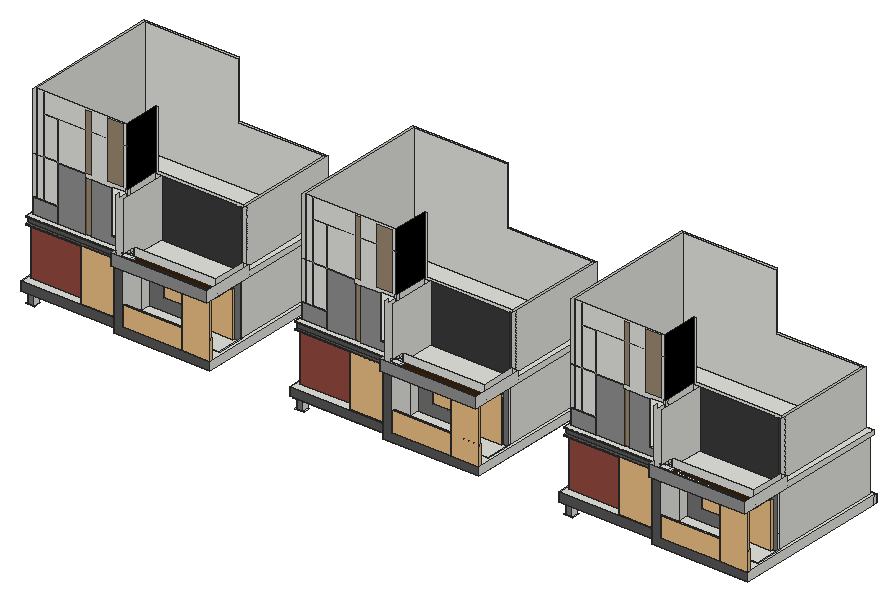
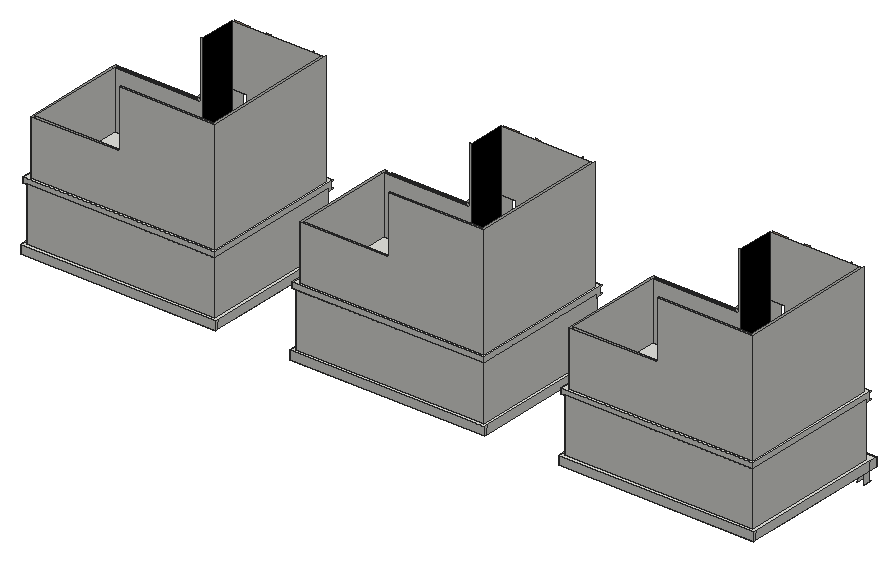
# SketchUp Ruby script. Lengths in inches.
U = 1.inch
M = Sketchup.active_model
def pt(a) = Geom::Point3d.new(a.map { |v| v * U })
def face(e, loops, mat)
  f = e.add_face(loops[0].map { |a| pt(a) })
  loops[1..].each { |l| e.add_face(l.map { |a| pt(a) }).erase! }
  f.material = f.back_material = mat if mat
  f
end
# faces: each face lists its corners as indices into pts; further lists are holes
def faces(e, pts, list, mat = nil) = list.each { |f| face(e, (f[0].is_a?(Array) ? f : [f]).map { |l| l.map { |i| pts[i] } }, mat) }
# xy, xz, yz: faces in a plane at the given z, y or x. An outline is a flat list of corners, or four numbers for a rectangle; further outlines are holes
def ring(l) = l.size == 4 ? [[l[0], l[1]], [l[2], l[1]], [l[2], l[3]], [l[0], l[3]]] : l.each_slice(2).to_a
def flat(e, list, mat, &to3) = list.each { |f| face(e, (f[0].is_a?(Array) ? f : [f]).map { |l| ring(l).map { |u, v| to3.(u, v) } }, mat) }
def xy(e, z, list, mat = nil) = flat(e, list, mat) { |x, y| [x, y, z] }
def xz(e, y, list, mat = nil) = flat(e, list, mat) { |x, z| [x, y, z] }
def yz(e, x, list, mat = nil) = flat(e, list, mat) { |y, z| [x, y, z] }
def lines(e, pts, list) = list.each { |a, b| e.add_line(pt(pts[a]), pt(pts[b])) }
# prism: a flat outline (further loops are holes) pulled along v
def prism(e, loops, v, mat = nil)
  f = face(e, loops, mat); d = Geom::Vector3d.new(v.map { |x| x * U })
  f.pushpull(f.normal.samedirection?(d) ? d.length : -d.length)
end
def box(e, o, s, mat = nil) = prism(e, [[o, [o[0] + s[0], o[1], o[2]], [o[0] + s[0], o[1] + s[1], o[2]], [o[0], o[1] + s[1], o[2]]]], [0, 0, s[2]], mat)
def at(x, y, z, deg = 0) = Geom::Transformation.translation(pt([x, y, z])) * Geom::Transformation.rotation(ORIGIN, Z_AXIS, deg.degrees)
def axes(o, x, y, z) = Geom::Transformation.new([*x, 0, *y, 0, *z, 0, *pt(o).to_a, 1])
def part(name) = M.definitions.add(name)
# library, detail: a bought-in or finely detailed component or shape, given as its bounding box
def library(name, o, s) = part(name).tap { |d| box(d.entities, o, s) }
def detail(e, o, s) = box(e.add_group.entities, o, s)
def put(e, d, t, mat = nil) = e.add_instance(d, t).tap { |i| i.material = mat if mat }
def group(e, t, mat = nil) = e.add_group.tap { |g| g.transformation = t; g.material = mat if mat }.entities
root = M.entities
M.materials.add("[Brick Antique 01]").color = [145, 73, 63]
M.materials.add("[Color C02]").color = [132, 106, 79]
M.materials["[Color C02]"].alpha = 0.77
M.materials.add("[Color C08]").color = [58, 29, 0]
M.materials.add("[Color M00]").color = [255, 255, 255]
M.materials.add("[Color M04]").color = [142, 142, 142]
M.materials.add("[Color M05]1").color = [114, 114, 114]
M.materials.add("[Color M06]1").color = [86, 86, 86]
M.materials.add("[Color M07]").color = [58, 58, 58]
M.materials.add("[Color M09]").color = [0, 0, 0]
c1 = library("door (1)",[38.93,25.48,0],[40,9.94,82.68])
c2 = library("JALI+PATTERN-03",[8.875,53.125,6.4375],[86,1,53.5])
c3 = library("Glass Railing",[0,0,0],[139.5,4.76,42])
c4 = library("Group\#2",[0,0,0],[40.6875,0.85,78])
c5 = library("3 door",[0,0,0],[74.8,3.9375,43.31])
c6 = library("Klein+raam",[128.36,12.7,0],[19.68,5.51,55.12])
xy(root,100.27,[[78.07,275.67,96.01,278.1],[641.2,275.67,659.14,278.1],[1204.32,275.67,1222.26,278.1],[78.07,278.1,80.51,291.17],[93.57,278.1,96.01,291.17],
  [641.2,278.1,643.64,291.17],[656.7,278.1,659.14,291.17],[1204.32,278.1,1206.76,291.17],[1219.82,278.1,1222.26,291.17]])
xy(root,126,[[281.09,252.1,482.625,278.1],[844.22,252.1,1045.75,278.1],[1407.34,252.1,1608.875,278.1],[73.5,267.1,79.84,284.83],[80.51,267.1,93.57,278.1],
  [280.26,267.1,281.09,278.1],[636.625,267.1,642.97,284.83],[643.64,267.1,656.7,278.1],[843.39,267.1,844.22,278.1],[1199.75,267.1,1206.09,284.83],
  [1206.76,267.1,1219.82,278.1],[1406.51,267.1,1407.34,278.1],[80.51,278.1,93.57,291.17],[280.26,278.1,295.26,291.17],[458.89,278.1,476.45,291.17],
  [643.64,278.1,656.7,291.17],[843.39,278.1,858.39,291.17],[1022.01,278.1,1039.57,291.17],[1206.76,278.1,1219.82,291.17],[1406.51,278.1,1421.51,291.17],
  [1585.14,278.1,1602.7,291.17],[73.5,284.83,79.84,498.32],[636.625,284.83,642.97,498.32],[1199.75,284.83,1206.09,498.32],[179.62,302.39,179.62,312.08,453.43,312.08,453.43,454.58,461.55,454.58,461.55,302.39],
  [742.74,302.39,742.74,312.08,1016.55,312.08,1016.55,454.58,1024.68,454.58,1024.68,302.39],[1305.87,302.39,1305.87,312.08,1579.68,312.08,1579.68,454.58,1587.8,454.58,1587.8,302.39],[73.5,498.32,79.84,581.15],[79.84,498.32,399.1,506.7],[399.1,498.32,482.625,581.15],
  [636.625,498.32,642.97,581.15],[642.97,498.32,962.22,506.7],[962.22,498.32,1045.75,581.15],[1199.75,498.32,1206.09,581.15],[1206.09,498.32,1525.35,506.7],
  [1525.35,498.32,1608.875,581.15],[79.84,506.7,399.1,581.15],[642.97,506.7,962.22,581.15],[1206.09,506.7,1525.35,581.15],[73.5,581.15,482.625,587.49],
  [636.625,581.15,1045.75,587.49],[1199.75,581.15,1608.875,587.49]])
xy(root,126,[[[79.84,267.1,79.84,498.32,482.625,498.32,482.625,278.1,476.45,278.1,476.45,291.17,458.89,291.17,458.89,278.1,295.26,278.1,295.26,291.17,280.26,291.17,280.26,267.1,93.57,267.1,93.57,291.17,80.51,291.17,80.51,267.1],[179.62,302.39,461.55,302.39,461.55,454.58,453.43,454.58,453.43,312.08,179.62,312.08]],[[642.97,267.1,642.97,498.32,1045.75,498.32,1045.75,278.1,1039.57,278.1,1039.57,291.17,1022.01,291.17,1022.01,278.1,858.39,278.1,858.39,291.17,843.39,291.17,843.39,267.1,656.7,267.1,656.7,291.17,643.64,291.17,643.64,267.1],[742.74,302.39,1024.68,302.39,1024.68,454.58,1016.55,454.58,1016.55,312.08,742.74,312.08]],[[1206.09,267.1,1206.09,498.32,1608.875,498.32,1608.875,278.1,1602.7,278.1,1602.7,291.17,1585.14,291.17,1585.14,278.1,1421.51,278.1,1421.51,291.17,1406.51,291.17,1406.51,267.1,1219.82,267.1,1219.82,291.17,1206.76,291.17,1206.76,267.1],[1305.87,302.39,1587.8,302.39,1587.8,454.58,1579.68,454.58,1579.68,312.08,1305.87,312.08]]],"[Color C08]")
xy(root,136.5625,[[280.5,285.73,475,285.73,475,345.45,470.34,345.45,470.34,290.39,280.5,290.39],[843.63,285.73,1038.12,285.73,1038.12,345.45,1033.47,345.45,1033.47,290.39,843.63,290.39],[1406.75,285.73,1601.25,285.73,1601.25,345.45,1596.59,345.45,1596.59,290.39,1406.75,290.39],[85.78,290.39,273.94,290.39,273.94,352.02,397.6,352.02,397.6,384.7,458.6,384.7,458.6,352.02,470.34,352.02,470.34,575.2,85.78,575.2],[280.5,290.39,470.34,290.39,470.34,345.45,458.6,345.45,458.6,352.02,397.6,352.02,397.6,345.45,280.5,345.45],
  [648.91,290.39,837.07,290.39,837.07,352.02,960.73,352.02,960.73,384.7,1021.73,384.7,1021.73,352.02,1033.47,352.02,1033.47,575.2,648.91,575.2],[843.63,290.39,1033.47,290.39,1033.47,345.45,1021.73,345.45,1021.73,352.02,960.73,352.02,960.73,345.45,843.63,345.45],[1212.03,290.39,1400.19,290.39,1400.19,352.02,1523.85,352.02,1523.85,384.7,1584.85,384.7,1584.85,352.02,1596.59,352.02,1596.59,575.2,1212.03,575.2],[1406.75,290.39,1596.59,290.39,1596.59,345.45,1584.85,345.45,1584.85,352.02,1523.85,352.02,1523.85,345.45,1406.75,345.45],[397.6,352.02,458.6,384.7],
  [960.73,352.02,1021.73,384.7],[1523.85,352.02,1584.85,384.7]])
xy(root,143.5,[[299.15,252.1,482.625,252.1,482.625,587.49,73.5,587.49,73.5,267.1,281.09,267.1,281.09,285.73,280.5,285.73,280.5,290.39,196.14,290.39,196.14,285.73,81.13,285.73,81.13,579.86,475,579.86,475,285.73,299.15,285.73],[862.27,252.1,1045.75,252.1,1045.75,587.49,636.625,587.49,636.625,267.1,844.22,267.1,844.22,285.73,843.63,285.73,843.63,290.39,759.27,290.39,759.27,285.73,644.25,285.73,644.25,579.86,1038.12,579.86,1038.12,285.73,862.27,285.73],[1425.4,252.1,1608.875,252.1,1608.875,587.49,1199.75,587.49,1199.75,267.1,1407.34,267.1,1407.34,285.73,1406.75,285.73,1406.75,290.39,1322.39,290.39,1322.39,285.73,1207.38,285.73,1207.38,579.86,1601.25,579.86,1601.25,285.73,1425.4,285.73],[281.09,278.1,299.15,285.73],[844.22,278.1,862.27,285.73],
  [1407.34,278.1,1425.4,285.73],[281.09,285.73,299.15,300.85],[844.22,285.73,862.27,300.85],[1407.34,285.73,1425.4,300.85]])
xy(root,160.79,[[311.14,345.45,359.51,384.7],[874.26,345.45,922.64,384.7],[1437.39,345.45,1485.76,384.7]])
xy(root,172.5,[[244.32,290.39,280.5,295.7],[807.44,290.39,843.63,295.7],[1370.57,290.39,1406.75,295.7]])
xy(root,228.23,[[311.14,345.45,359.51,384.7],[874.26,345.45,922.64,384.7],[1437.39,345.45,1485.76,384.7]])
xy(root,228.63,[[244.32,290.39,280.5,295.7],[807.44,290.39,843.63,295.7],[1370.57,290.39,1406.75,295.7]])
xy(root,230.0625,[[397.6,345.45,458.6,384.7],[960.73,345.45,1021.73,384.7],[1523.85,345.45,1584.85,384.7]])
xy(root,250.75,[[81.13,271.23,81.13,285.73,280.5,285.73,280.5,345.45,281.09,345.45,281.09,271.23],[644.25,271.23,644.25,285.73,843.63,285.73,843.63,345.45,844.22,345.45,844.22,271.23],[1207.38,271.23,1207.38,285.73,1406.75,285.73,1406.75,345.45,1407.34,345.45,1407.34,271.23],[196.14,285.73,280.5,290.39],[759.27,285.73,843.63,290.39],
  [1322.39,285.73,1406.75,290.39]])
xy(root,252.73,[[81.13,271.23,281.09,277.85],[644.25,271.23,844.22,277.85],[1207.38,271.23,1407.34,277.85]],"[Color M06]1")
xy(root,256.5625,[[281.09,243.1,299.15,252.1],[299.15,243.1,482.625,256.29],[844.22,243.1,862.27,252.1],[862.27,243.1,1045.75,256.29],[1407.34,243.1,1425.4,252.1],
  [1425.4,243.1,1608.875,256.29],[281.09,252.1,299.15,256.29],[844.22,252.1,862.27,256.29],[1407.34,252.1,1425.4,256.29],[299.15,256.29,482.625,271.23],
  [862.27,256.29,1045.75,271.23],[1425.4,256.29,1608.875,271.23],[281.09,271.23,299.15,300.85],[844.22,271.23,862.27,300.85],[1407.34,271.23,1425.4,300.85],
  [[81.13,285.73,81.13,579.86,475,579.86,475,345.45,280.5,345.45,280.5,285.73],[85.78,290.39,273.94,290.39,273.94,352.02,470.34,352.02,470.34,575.2,85.78,575.2]],[[644.25,285.73,644.25,579.86,1038.12,579.86,1038.12,345.45,843.63,345.45,843.63,285.73],[648.91,290.39,837.07,290.39,837.07,352.02,1033.47,352.02,1033.47,575.2,648.91,575.2]],[[1207.38,285.73,1207.38,579.86,1601.25,579.86,1601.25,345.45,1406.75,345.45,1406.75,285.73],[1212.03,290.39,1400.19,290.39,1400.19,352.02,1596.59,352.02,1596.59,575.2,1212.03,575.2]],[475,345.45,482.625,579.86],[1038.12,345.45,1045.75,579.86],
  [1601.25,345.45,1608.875,579.86]])
xy(root,256.5625,[[[299.15,271.23,299.15,300.85,281.09,300.85,281.09,345.45,482.625,345.45,482.625,271.23],[310.37,279.3,449.37,279.3,449.37,282.49,313.05,282.49,313.05,328.87,310.37,328.87]],[[862.27,271.23,862.27,300.85,844.22,300.85,844.22,345.45,1045.75,345.45,1045.75,271.23],[873.49,279.3,1012.49,279.3,1012.49,282.49,876.18,282.49,876.18,328.87,873.49,328.87]],[[1425.4,271.23,1425.4,300.85,1407.34,300.85,1407.34,345.45,1608.875,345.45,1608.875,271.23],[1436.62,279.3,1575.62,279.3,1575.62,282.49,1439.3,282.49,1439.3,328.87,1436.62,328.87]]],"[Color C08]")
xy(root,256.5625,[[310.37,279.3,310.37,328.87,313.05,328.87,313.05,282.49,449.37,282.49,449.37,279.3],[873.49,279.3,873.49,328.87,876.18,328.87,876.18,282.49,1012.49,282.49,1012.49,279.3],[1436.62,279.3,1436.62,328.87,1439.3,328.87,1439.3,282.49,1575.62,282.49,1575.62,279.3]],"[Color M00]")
xy(root,262.5625,[[281.09,271.23,299.15,283.04],[844.22,271.23,862.27,283.04],[1407.34,271.23,1425.4,283.04],[285.28,283.04,299.15,287.65],[299.15,283.04,470.0625,283.04,470.0625,354.29,465.45,354.29,465.45,287.65,299.15,287.65],
  [848.4,283.04,862.27,287.65],[862.27,283.04,1033.1875,283.04,1033.1875,354.29,1028.58,354.29,1028.58,287.65,862.27,287.65],[1411.53,283.04,1425.4,287.65],[1425.4,283.04,1596.3125,283.04,1596.3125,354.29,1591.7,354.29,1591.7,287.65,1425.4,287.65],[90.67,287.65,280.83,287.65,280.83,362.98,465.45,362.98,465.45,570.3125,90.67,570.3125],
  [285.28,287.65,299.15,354.29],[299.15,287.65,465.45,354.29],[653.8,287.65,843.96,287.65,843.96,362.98,1028.58,362.98,1028.58,570.3125,653.8,570.3125],[848.4,287.65,862.27,354.29],[862.27,287.65,1028.58,354.29],
  [1216.92,287.65,1407.08,287.65,1407.08,362.98,1591.7,362.98,1591.7,570.3125,1216.92,570.3125],[1411.53,287.65,1425.4,354.29],[1425.4,287.65,1591.7,354.29]])
xy(root,265.59,[[81.13,271.23,281.09,277.85],[644.25,271.23,844.22,277.85],[1207.38,271.23,1407.34,277.85]],"[Color M06]1")
xy(root,267.5625,[[81.13,271.23,281.09,271.23,281.09,283.04,86.0625,283.04,86.0625,574.92,470.0625,574.92,470.0625,354.29,482.625,354.29,482.625,579.86,81.13,579.86],[644.25,271.23,844.22,271.23,844.22,283.04,649.1875,283.04,649.1875,574.92,1033.1875,574.92,1033.1875,354.29,1045.75,354.29,1045.75,579.86,644.25,579.86],[1207.38,271.23,1407.34,271.23,1407.34,283.04,1212.3125,283.04,1212.3125,574.92,1596.3125,574.92,1596.3125,354.29,1608.875,354.29,1608.875,579.86,1207.38,579.86]])
xz(root,243.1,[[281.09,256.5625,482.625,279.5625],[844.22,256.5625,1045.75,279.5625],[1407.34,256.5625,1608.875,279.5625]],"[Color M04]")
xz(root,252.1,[[281.09,126,482.625,126,482.625,143.5,299.15,143.5,299.15,256.5625,281.09,256.5625],[844.22,126,1045.75,126,1045.75,143.5,862.27,143.5,862.27,256.5625,844.22,256.5625],[1407.34,126,1608.875,126,1608.875,143.5,1425.4,143.5,1425.4,256.5625,1407.34,256.5625]],"[Color M06]1")
xz(root,267.1,[[73.5,126,281.09,143.5],[636.625,126,844.22,143.5],[1199.75,126,1407.34,143.5]],"[Color M06]1")
xz(root,271.23,[[281.09,256.5625,299.15,262.5625],[844.22,256.5625,862.27,262.5625],[1407.34,256.5625,1425.4,262.5625]])
xz(root,271.23,[[81.13,250.75,281.09,252.73],[644.25,250.75,844.22,252.73],[1207.38,250.75,1407.34,252.73],[81.13,265.59,281.09,267.5625],[644.25,265.59,844.22,267.5625],
  [1207.38,265.59,1407.34,267.5625]],"[Color M06]1")
xz(root,277.85,[[81.13,252.73,281.09,265.59],[644.25,252.73,844.22,265.59],[1207.38,252.73,1407.34,265.59]],"[Color M06]1")
xz(root,278.1,[[80.51,100.27,93.57,126],[643.64,100.27,656.7,126],[1206.76,100.27,1219.82,126]],"[Color M05]1")
xz(root,283.04,[[281.09,262.5625,285.28,382.5625],[299.15,262.5625,470.0625,279.5625],[844.22,262.5625,848.4,382.5625],[862.27,262.5625,1033.1875,279.5625],[1407.34,262.5625,1411.53,382.5625],
  [1425.4,262.5625,1596.3125,279.5625]])
xz(root,283.04,[[[138.73,267.5625,140.54,267.5625,140.54,380.6,196.53,380.6,196.53,382.5625,140.54,382.5625,140.54,462.57,198.84,462.57,198.84,382.5625,210.82,382.5625,210.82,462.57,243.69,462.57,243.69,382.5625,277.35,382.5625,277.35,462.57,285.28,462.57,285.28,463.9375,277.35,463.9375,277.35,502.5625,243.69,502.5625,243.69,463.9375,210.82,463.9375,210.82,502.5625,198.84,502.5625,198.84,463.9375,111.72,463.9375,111.72,502.5625,109.54,502.5625,109.54,382.5625,86.0625,382.5625,86.0625,380.6,109.54,380.6,109.54,301.46,86.0625,301.46,86.0625,299.14,138.73,299.14],[111.72,382.5625,138.73,462.57],[111.72,301.46,138.73,380.6]],[198.84,267.5625,210.82,374],[[701.85,267.5625,703.67,267.5625,703.67,380.6,759.65,380.6,759.65,382.5625,703.67,382.5625,703.67,462.57,761.97,462.57,761.97,382.5625,773.94,382.5625,773.94,462.57,806.82,462.57,806.82,382.5625,840.48,382.5625,840.48,462.57,848.4,462.57,848.4,463.9375,840.48,463.9375,840.48,502.5625,806.82,502.5625,806.82,463.9375,773.94,463.9375,773.94,502.5625,761.97,502.5625,761.97,463.9375,674.85,463.9375,674.85,502.5625,672.66,502.5625,672.66,382.5625,649.1875,382.5625,649.1875,380.6,672.66,380.6,672.66,301.46,649.1875,301.46,649.1875,299.14,701.85,299.14],[674.85,382.5625,701.85,462.57],[674.85,301.46,701.85,380.6]],[761.97,267.5625,773.94,374],[[1264.98,267.5625,1266.79,267.5625,1266.79,380.6,1322.78,380.6,1322.78,382.5625,1266.79,382.5625,1266.79,462.57,1325.09,462.57,1325.09,382.5625,1337.07,382.5625,1337.07,462.57,1369.94,462.57,1369.94,382.5625,1403.6,382.5625,1403.6,462.57,1411.53,462.57,1411.53,463.9375,1403.6,463.9375,1403.6,502.5625,1369.94,502.5625,1369.94,463.9375,1337.07,463.9375,1337.07,502.5625,1325.09,502.5625,1325.09,463.9375,1237.97,463.9375,1237.97,502.5625,1235.79,502.5625,1235.79,382.5625,1212.3125,382.5625,1212.3125,380.6,1235.79,380.6,1235.79,301.46,1212.3125,301.46,1212.3125,299.14,1264.98,299.14],[1237.97,382.5625,1264.98,462.57],[1237.97,301.46,1264.98,380.6]],
  [1325.09,267.5625,1337.07,374]],"[Color C02]")
xz(root,283.04,[[86.0625,267.5625,138.73,299.14],[140.54,267.5625,198.84,267.5625,198.84,374,196.53,374,196.53,380.6,140.54,380.6],[210.82,267.5625,281.09,267.5625,281.09,283.9375,249.28,283.9375,249.28,374,210.82,374],[649.1875,267.5625,701.85,299.14],[703.67,267.5625,761.97,267.5625,761.97,374,759.65,374,759.65,380.6,703.67,380.6],
  [773.94,267.5625,844.22,267.5625,844.22,283.9375,812.4,283.9375,812.4,374,773.94,374],[1212.3125,267.5625,1264.98,299.14],[1266.79,267.5625,1325.09,267.5625,1325.09,374,1322.78,374,1322.78,380.6,1266.79,380.6],[1337.07,267.5625,1407.34,267.5625,1407.34,283.9375,1375.53,283.9375,1375.53,374,1337.07,374]],"[Color M04]")
xz(root,285.73,[[280.5,136.5625,399.1,143.5],[399.1,136.5625,475,143.5],[843.63,136.5625,962.22,143.5],[962.22,136.5625,1038.12,143.5],[1406.75,136.5625,1525.35,143.5],
  [1525.35,136.5625,1601.25,143.5],[81.13,250.75,280.5,256.5625],[644.25,250.75,843.63,256.5625],[1207.38,250.75,1406.75,256.5625]])
xz(root,285.73,[[81.13,143.5,196.14,250.75],[644.25,143.5,759.27,250.75],[1207.38,143.5,1322.39,250.75]],"[Brick Antique 01]")
xz(root,287.65,[[90.67,262.5625,90.67,502.5625,280.83,502.5625,280.83,374,249.28,374,249.28,283.9375,280.83,283.9375,280.83,262.5625],[653.8,262.5625,653.8,502.5625,843.96,502.5625,843.96,374,812.4,374,812.4,283.9375,843.96,283.9375,843.96,262.5625],[1216.92,262.5625,1216.92,502.5625,1407.08,502.5625,1407.08,374,1375.53,374,1375.53,283.9375,1407.08,283.9375,1407.08,262.5625]])
xz(root,290.39,[[196.14,143.5,280.5,143.5,280.5,172.5,244.32,172.5,244.32,228.63,280.5,228.63,280.5,250.75,196.14,250.75],[759.27,143.5,843.63,143.5,843.63,172.5,807.44,172.5,807.44,228.63,843.63,228.63,843.63,250.75,759.27,250.75],[1322.39,143.5,1406.75,143.5,1406.75,172.5,1370.57,172.5,1370.57,228.63,1406.75,228.63,1406.75,250.75,1322.39,250.75]])
xz(root,295.7,[[244.32,172.5,280.5,228.63],[807.44,172.5,843.63,228.63],[1370.57,172.5,1406.75,228.63]],"[Color M09]")
xz(root,300.85,[[281.09,143.5,299.15,256.5625],[844.22,143.5,862.27,256.5625],[1407.34,143.5,1425.4,256.5625]])
xz(root,345.45,[[470.34,136.5625,475,256.5625],[1033.47,136.5625,1038.12,256.5625],[1596.59,136.5625,1601.25,256.5625],[280.5,250.75,281.09,256.5625],[843.63,250.75,844.22,256.5625],
  [1406.75,250.75,1407.34,256.5625]])
xz(root,345.45,[[[280.5,136.5625,397.6,136.5625,397.6,230.0625,458.6,230.0625,458.6,136.5625,470.34,136.5625,470.34,256.5625,281.09,256.5625,281.09,250.75,280.5,250.75],[311.14,160.79,359.51,228.23]],[[843.63,136.5625,960.73,136.5625,960.73,230.0625,1021.73,230.0625,1021.73,136.5625,1033.47,136.5625,1033.47,256.5625,844.22,256.5625,844.22,250.75,843.63,250.75],[874.26,160.79,922.64,228.23]],[[1406.75,136.5625,1523.85,136.5625,1523.85,230.0625,1584.85,230.0625,1584.85,136.5625,1596.59,136.5625,1596.59,256.5625,1407.34,256.5625,1407.34,250.75,1406.75,250.75],[1437.39,160.79,1485.76,228.23]]],"[Color M05]1")
xz(root,352.02,[[273.94,136.5625,280.5,256.5625],[837.07,136.5625,843.63,256.5625],[1400.19,136.5625,1406.75,256.5625]])
xz(root,352.02,[[280.5,136.5625,470.34,256.5625],[843.63,136.5625,1033.47,256.5625],[1406.75,136.5625,1596.59,256.5625]],"[Color M09]")
xz(root,354.29,[[285.28,262.5625,299.15,382.5625],[848.4,262.5625,862.27,382.5625],[1411.53,262.5625,1425.4,382.5625],[470.0625,267.5625,482.625,279.5625],[1033.1875,267.5625,1045.75,279.5625],
  [1596.3125,267.5625,1608.875,279.5625]])
xz(root,354.29,[[299.15,262.5625,465.45,262.5625,465.45,381.5,455.68,381.5,455.68,382.5625,299.15,382.5625],[465.45,262.5625,470.0625,382.5625],[862.27,262.5625,1028.58,262.5625,1028.58,381.5,1018.8,381.5,1018.8,382.5625,862.27,382.5625],[1028.58,262.5625,1033.1875,382.5625],[1425.4,262.5625,1591.7,262.5625,1591.7,381.5,1581.93,381.5,1581.93,382.5625,1425.4,382.5625],
  [1591.7,262.5625,1596.3125,382.5625]],"[Color M07]")
xz(root,362.98,[[280.83,262.5625,280.83,502.5625,285.28,502.5625,285.28,382.5625,465.45,382.5625,465.45,262.5625],[843.96,262.5625,843.96,502.5625,848.4,502.5625,848.4,382.5625,1028.58,382.5625,1028.58,262.5625],[1407.08,262.5625,1407.08,502.5625,1411.53,502.5625,1411.53,382.5625,1591.7,382.5625,1591.7,262.5625]])
xz(root,384.7,[[397.6,136.5625,458.6,230.0625],[960.73,136.5625,1021.73,230.0625],[1523.85,136.5625,1584.85,230.0625],[311.14,160.79,359.51,228.23],[874.26,160.79,922.64,228.23],
  [1437.39,160.79,1485.76,228.23]])
xz(root,570.3125,[[90.67,262.5625,465.45,262.5625,465.45,382.5625,285.28,382.5625,285.28,502.5625,90.67,502.5625],[653.8,262.5625,1028.58,262.5625,1028.58,382.5625,848.4,382.5625,848.4,502.5625,653.8,502.5625],[1216.92,262.5625,1591.7,262.5625,1591.7,382.5625,1411.53,382.5625,1411.53,502.5625,1216.92,502.5625]])
xz(root,574.92,[[86.0625,267.5625,86.0625,502.5625,285.28,502.5625,285.28,382.5625,470.0625,382.5625,470.0625,267.5625],[649.1875,267.5625,649.1875,502.5625,848.4,502.5625,848.4,382.5625,1033.1875,382.5625,1033.1875,267.5625],[1212.3125,267.5625,1212.3125,502.5625,1411.53,502.5625,1411.53,382.5625,1596.3125,382.5625,1596.3125,267.5625]])
xz(root,575.2,[[85.78,136.5625,470.34,256.5625],[648.91,136.5625,1033.47,256.5625],[1212.03,136.5625,1596.59,256.5625]])
xz(root,579.86,[[81.13,143.5,475,256.5625],[644.25,143.5,1038.12,256.5625],[1207.38,143.5,1601.25,256.5625],[81.13,256.5625,482.625,267.5625],[644.25,256.5625,1045.75,267.5625],
  [1207.38,256.5625,1608.875,267.5625]])
xz(root,587.49,[[73.5,126,482.625,143.5],[636.625,126,1045.75,143.5],[1199.75,126,1608.875,143.5]])
yz(root,73.5,[[267.1,126,284.83,143.5],[284.83,126,581.15,143.5],[581.15,126,587.49,143.5]])
yz(root,80.51,[[278.1,100.27,291.17,126]])
yz(root,81.13,[[285.73,143.5,579.86,256.5625],[271.23,250.75,271.23,252.73,277.85,252.73,277.85,265.59,271.23,265.59,271.23,267.5625,579.86,267.5625,579.86,256.5625,285.73,256.5625,285.73,250.75]])
yz(root,85.78,[[290.39,136.5625,575.2,256.5625]])
yz(root,86.0625,[[283.04,267.5625,574.92,502.5625]])
yz(root,90.67,[[287.65,262.5625,570.3125,502.5625]])
yz(root,93.57,[[278.1,100.27,291.17,126]])
yz(root,196.14,[[285.73,143.5,290.39,250.75]])
yz(root,244.32,[[290.39,172.5,295.7,228.63]])
yz(root,280.5,[[285.73,136.5625,290.39,143.5],[290.39,136.5625,345.45,136.5625,345.45,250.75,290.39,250.75,290.39,228.63,295.7,228.63,295.7,172.5,290.39,172.5],[285.73,250.75,290.39,256.5625],[290.39,250.75,345.45,256.5625]])
yz(root,280.83,[[287.65,262.5625,362.98,502.5625]],"[Color M09]")
yz(root,281.09,[[252.1,126,252.1,256.5625,256.29,256.5625,256.29,382.5625,264.41,382.5625,264.41,374,283.04,374,283.04,267.5625,271.23,267.5625,271.23,265.59,277.85,265.59,277.85,262.5625,271.23,262.5625,271.23,256.5625,277.85,256.5625,277.85,252.73,271.23,252.73,271.23,250.75,300.85,250.75,300.85,143.5,267.1,143.5,267.1,126],[267.1,126,278.1,143.5],[271.23,250.75,300.85,250.75,300.85,256.5625,277.85,256.5625,277.85,252.73,271.23,252.73],[300.85,250.75,345.45,256.5625],[243.1,256.5625,256.29,279.5625],
  [271.23,256.5625,277.85,262.5625],[277.85,262.5625,277.85,265.59,271.23,265.59,271.23,267.5625,283.04,267.5625,283.04,262.5625]])
yz(root,285.28,[[283.04,262.5625,287.65,382.5625],[287.65,262.5625,354.29,382.5625]])
yz(root,299.15,[[252.1,143.5,300.85,256.5625],[283.04,262.5625,354.29,262.5625,354.29,382.5625,256.29,382.5625,256.29,279.5625,283.04,279.5625]])
yz(root,311.14,[[345.45,160.79,384.7,228.23]])
yz(root,359.51,[[345.45,160.79,384.7,228.23]])
yz(root,397.6,[[345.45,136.5625,384.7,230.0625]])
yz(root,458.6,[[345.45,136.5625,384.7,230.0625]])
yz(root,465.45,[[362.98,262.5625,570.3125,382.5625]])
yz(root,470.0625,[[283.04,262.5625,354.29,279.5625],[354.29,267.5625,362.98,382.5625],[362.98,267.5625,574.92,382.5625]])
yz(root,470.34,[[352.02,136.5625,575.2,256.5625]])
yz(root,475,[[285.73,136.5625,345.45,143.5],[345.45,143.5,579.86,256.5625]])
yz(root,482.625,[[252.1,126,581.15,143.5],[581.15,126,587.49,143.5],[243.1,256.5625,579.86,256.5625,579.86,267.5625,354.29,267.5625,354.29,279.5625,243.1,279.5625]])
yz(root,636.625,[[267.1,126,284.83,143.5],[284.83,126,581.15,143.5],[581.15,126,587.49,143.5]])
yz(root,643.64,[[278.1,100.27,291.17,126]])
yz(root,644.25,[[285.73,143.5,579.86,256.5625],[271.23,250.75,271.23,252.73,277.85,252.73,277.85,265.59,271.23,265.59,271.23,267.5625,579.86,267.5625,579.86,256.5625,285.73,256.5625,285.73,250.75]])
yz(root,648.91,[[290.39,136.5625,575.2,256.5625]])
yz(root,649.1875,[[283.04,267.5625,574.92,502.5625]])
yz(root,653.8,[[287.65,262.5625,570.3125,502.5625]])
yz(root,656.7,[[278.1,100.27,291.17,126]])
yz(root,759.27,[[285.73,143.5,290.39,250.75]])
yz(root,807.44,[[290.39,172.5,295.7,228.63]])
yz(root,843.63,[[285.73,136.5625,290.39,143.5],[290.39,136.5625,345.45,136.5625,345.45,250.75,290.39,250.75,290.39,228.63,295.7,228.63,295.7,172.5,290.39,172.5],[285.73,250.75,290.39,256.5625],[290.39,250.75,345.45,256.5625]])
yz(root,843.96,[[287.65,262.5625,362.98,502.5625]],"[Color M09]")
yz(root,844.22,[[252.1,126,252.1,256.5625,256.29,256.5625,256.29,382.5625,264.41,382.5625,264.41,374,283.04,374,283.04,267.5625,271.23,267.5625,271.23,265.59,277.85,265.59,277.85,262.5625,271.23,262.5625,271.23,256.5625,277.85,256.5625,277.85,252.73,271.23,252.73,271.23,250.75,300.85,250.75,300.85,143.5,267.1,143.5,267.1,126],[267.1,126,278.1,143.5],[271.23,250.75,300.85,250.75,300.85,256.5625,277.85,256.5625,277.85,252.73,271.23,252.73],[300.85,250.75,345.45,256.5625],[243.1,256.5625,256.29,279.5625],
  [271.23,256.5625,277.85,262.5625],[277.85,262.5625,277.85,265.59,271.23,265.59,271.23,267.5625,283.04,267.5625,283.04,262.5625]])
yz(root,848.4,[[283.04,262.5625,287.65,382.5625],[287.65,262.5625,354.29,382.5625]])
yz(root,862.27,[[252.1,143.5,300.85,256.5625],[283.04,262.5625,354.29,262.5625,354.29,382.5625,256.29,382.5625,256.29,279.5625,283.04,279.5625]])
yz(root,874.26,[[345.45,160.79,384.7,228.23]])
yz(root,922.64,[[345.45,160.79,384.7,228.23]])
yz(root,960.73,[[345.45,136.5625,384.7,230.0625]])
yz(root,1021.73,[[345.45,136.5625,384.7,230.0625]])
yz(root,1028.58,[[362.98,262.5625,570.3125,382.5625]])
yz(root,1033.1875,[[283.04,262.5625,354.29,279.5625],[354.29,267.5625,362.98,382.5625],[362.98,267.5625,574.92,382.5625]])
yz(root,1033.47,[[352.02,136.5625,575.2,256.5625]])
yz(root,1038.12,[[285.73,136.5625,345.45,143.5],[345.45,143.5,579.86,256.5625]])
yz(root,1045.75,[[252.1,126,581.15,143.5],[581.15,126,587.49,143.5],[243.1,256.5625,579.86,256.5625,579.86,267.5625,354.29,267.5625,354.29,279.5625,243.1,279.5625]])
yz(root,1199.75,[[267.1,126,284.83,143.5],[284.83,126,581.15,143.5],[581.15,126,587.49,143.5]])
yz(root,1206.76,[[278.1,100.27,291.17,126]])
yz(root,1207.38,[[285.73,143.5,579.86,256.5625],[271.23,250.75,271.23,252.73,277.85,252.73,277.85,265.59,271.23,265.59,271.23,267.5625,579.86,267.5625,579.86,256.5625,285.73,256.5625,285.73,250.75]])
yz(root,1212.03,[[290.39,136.5625,575.2,256.5625]])
yz(root,1212.3125,[[283.04,267.5625,574.92,502.5625]])
yz(root,1216.92,[[287.65,262.5625,570.3125,502.5625]])
yz(root,1219.82,[[278.1,100.27,291.17,126]])
yz(root,1322.39,[[285.73,143.5,290.39,250.75]])
yz(root,1370.57,[[290.39,172.5,295.7,228.63]])
yz(root,1406.75,[[285.73,136.5625,290.39,143.5],[290.39,136.5625,345.45,136.5625,345.45,250.75,290.39,250.75,290.39,228.63,295.7,228.63,295.7,172.5,290.39,172.5],[285.73,250.75,290.39,256.5625],[290.39,250.75,345.45,256.5625]])
yz(root,1407.08,[[287.65,262.5625,362.98,502.5625]],"[Color M09]")
yz(root,1407.34,[[252.1,126,252.1,256.5625,256.29,256.5625,256.29,382.5625,264.41,382.5625,264.41,374,283.04,374,283.04,267.5625,271.23,267.5625,271.23,265.59,277.85,265.59,277.85,262.5625,271.23,262.5625,271.23,256.5625,277.85,256.5625,277.85,252.73,271.23,252.73,271.23,250.75,300.85,250.75,300.85,143.5,267.1,143.5,267.1,126],[267.1,126,278.1,143.5],[271.23,250.75,300.85,250.75,300.85,256.5625,277.85,256.5625,277.85,252.73,271.23,252.73],[300.85,250.75,345.45,256.5625],[243.1,256.5625,256.29,279.5625],
  [271.23,256.5625,277.85,262.5625],[277.85,262.5625,277.85,265.59,271.23,265.59,271.23,267.5625,283.04,267.5625,283.04,262.5625]])
yz(root,1411.53,[[283.04,262.5625,287.65,382.5625],[287.65,262.5625,354.29,382.5625]])
yz(root,1425.4,[[252.1,143.5,300.85,256.5625],[283.04,262.5625,354.29,262.5625,354.29,382.5625,256.29,382.5625,256.29,279.5625,283.04,279.5625]])
yz(root,1437.39,[[345.45,160.79,384.7,228.23]])
yz(root,1485.76,[[345.45,160.79,384.7,228.23]])
yz(root,1523.85,[[345.45,136.5625,384.7,230.0625]])
yz(root,1584.85,[[345.45,136.5625,384.7,230.0625]])
yz(root,1591.7,[[362.98,262.5625,570.3125,382.5625]])
yz(root,1596.3125,[[283.04,262.5625,354.29,279.5625],[354.29,267.5625,362.98,382.5625],[362.98,267.5625,574.92,382.5625]])
yz(root,1596.59,[[352.02,136.5625,575.2,256.5625]])
yz(root,1601.25,[[285.73,136.5625,345.45,143.5],[345.45,143.5,579.86,256.5625]])
yz(root,1608.875,[[252.1,126,581.15,143.5],[581.15,126,587.49,143.5],[243.1,256.5625,579.86,256.5625,579.86,267.5625,354.29,267.5625,354.29,279.5625,243.1,279.5625]])
p = [[962.22,581.15,126],[962.22,581.15,136.5625],[642.97,581.15,126],[642.97,581.15,136.5625],[642.97,284.83,126],[642.97,284.83,136.5625],
  [1045.75,271.23,262.5625],[862.27,271.23,262.5625],[1033.1875,354.29,262.5625],[1045.75,354.29,262.5625],[1206.09,284.83,126],[1206.09,284.83,136.5625],
  [1525.35,581.15,126],[1525.35,581.15,136.5625],[1206.09,581.15,126],[1206.09,581.15,136.5625],[1608.875,271.23,262.5625],[1425.4,271.23,262.5625],
  [1596.3125,354.29,262.5625],[1608.875,354.29,262.5625],[470.0625,354.29,262.5625],[482.625,354.29,262.5625],[399.1,581.15,126],[399.1,581.15,136.5625],
  [79.84,581.15,126],[79.84,581.15,136.5625],[482.625,271.23,262.5625],[299.15,271.23,262.5625],[79.84,284.83,126],[79.84,284.83,136.5625]]
lines(root,p,[[0,1],[2,3],[4,5],[6,7],[8,9],[10,11],[12,13],[14,15],[16,17],[18,19],[20,21],[22,23],
  [24,25],[26,27],[28,29]])
put(root,c1,axes([901.36,312.625,136.5625],[1.525,0,0],[0,1.13,0],[0,0,1.13]))
put(root,c1,axes([338.24,312.625,136.5625],[1.525,0,0],[0,1.13,0],[0,0,1.13]))
put(root,c1,axes([1464.49,312.625,136.5625],[1.525,0,0],[0,1.13,0],[0,0,1.13]))
put(root,c2,axes([748.85,204.82,261.84],[0,0,-1.25],[0,1.25,0],[1.61807,0,0]))
put(root,c2,axes([185.73,204.82,261.84],[0,0,-1.25],[0,1.25,0],[1.61807,0,0]))
put(root,c2,axes([1311.98,204.82,261.84],[0,0,-1.25],[0,1.25,0],[1.61807,0,0]))
put(root,c3,axes([862.27,252.1,143.5],[1.31526,0,0],[0,1,0],[0,0,1]))
put(root,c3,axes([299.15,252.1,143.5],[1.31526,0,0],[0,1,0],[0,0,1]))
put(root,c4,axes([986.67,251.99,143.5],[1.452,0,0],[0,1.452,0],[0,0,1.452]))
put(root,c4,axes([423.55,251.99,143.5],[1.452,0,0],[0,1.452,0],[0,0,1.452]))
put(root,c3,axes([1425.4,252.1,143.5],[1.31526,0,0],[0,1,0],[0,0,1]))
put(root,c4,axes([1549.8,251.99,143.5],[1.452,0,0],[0,1.452,0],[0,0,1.452]))
put(root,c5,axes([874.26,345.45,228.23],[0,0,-0.90153],[0,1,0],[1.11702,0,0]))
put(root,c5,axes([311.14,345.45,228.23],[0,0,-0.90153],[0,1,0],[1.11702,0,0]))
put(root,c5,axes([1437.39,345.45,228.23],[0,0,-0.90153],[0,1,0],[1.11702,0,0]))
put(root,c6,axes([567.65,277.69,172.5],[1.86812,0,0],[0,1,0],[0,0,1]))
put(root,c6,axes([4.53,277.69,172.5],[1.86812,0,0],[0,1,0],[0,0,1]))
put(root,c6,axes([1130.78,277.69,172.5],[1.86812,0,0],[0,1,0],[0,0,1]))
